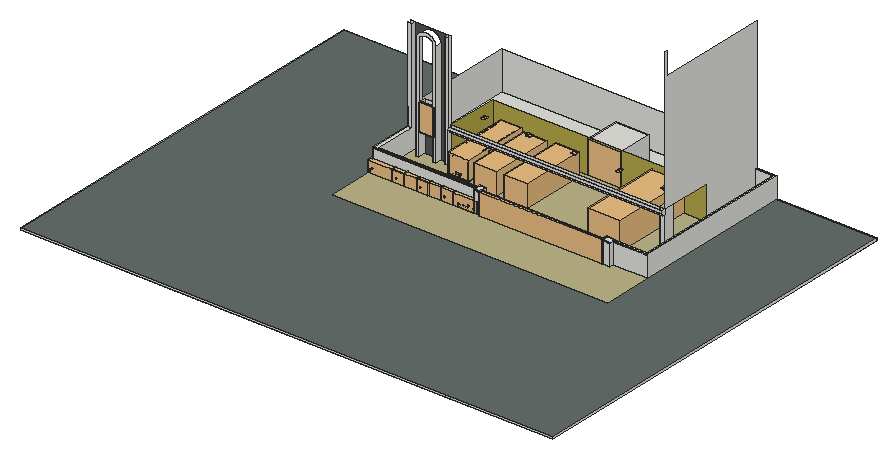
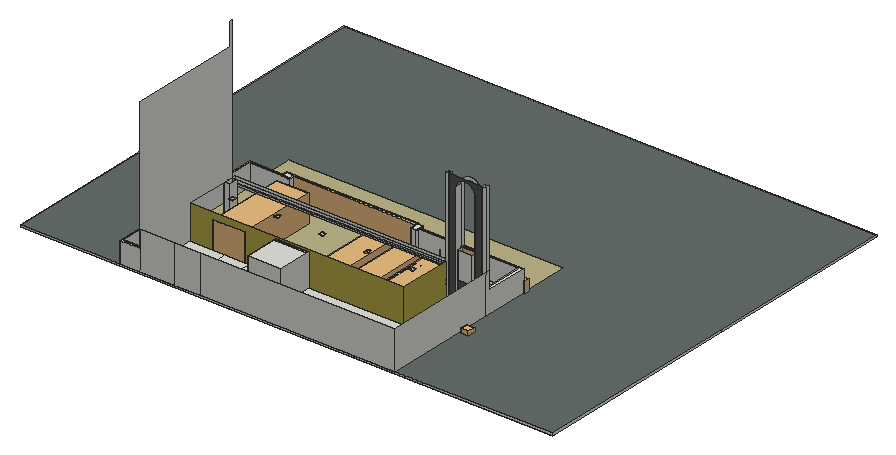
# SketchUp Ruby script. Lengths in inches.
U = 1.inch
M = Sketchup.active_model
def pt(a) = Geom::Point3d.new(a.map { |v| v * U })
def face(e, loops, mat)
  f = e.add_face(loops[0].map { |a| pt(a) })
  loops[1..].each { |l| e.add_face(l.map { |a| pt(a) }).erase! }
  f.material = f.back_material = mat if mat
  f
end
# faces: each face lists its corners as indices into pts; further lists are holes
def faces(e, pts, list, mat = nil) = list.each { |f| face(e, (f[0].is_a?(Array) ? f : [f]).map { |l| l.map { |i| pts[i] } }, mat) }
# xy, xz, yz: faces in a plane at the given z, y or x. An outline is a flat list of corners, or four numbers for a rectangle; further outlines are holes
def ring(l) = l.size == 4 ? [[l[0], l[1]], [l[2], l[1]], [l[2], l[3]], [l[0], l[3]]] : l.each_slice(2).to_a
def flat(e, list, mat, &to3) = list.each { |f| face(e, (f[0].is_a?(Array) ? f : [f]).map { |l| ring(l).map { |u, v| to3.(u, v) } }, mat) }
def xy(e, z, list, mat = nil) = flat(e, list, mat) { |x, y| [x, y, z] }
def xz(e, y, list, mat = nil) = flat(e, list, mat) { |x, z| [x, y, z] }
def yz(e, x, list, mat = nil) = flat(e, list, mat) { |y, z| [x, y, z] }
def lines(e, pts, list) = list.each { |a, b| e.add_line(pt(pts[a]), pt(pts[b])) }
# prism: a flat outline (further loops are holes) pulled along v
def prism(e, loops, v, mat = nil)
  f = face(e, loops, mat); d = Geom::Vector3d.new(v.map { |x| x * U })
  f.pushpull(f.normal.samedirection?(d) ? d.length : -d.length)
end
def box(e, o, s, mat = nil) = prism(e, [[o, [o[0] + s[0], o[1], o[2]], [o[0] + s[0], o[1] + s[1], o[2]], [o[0], o[1] + s[1], o[2]]]], [0, 0, s[2]], mat)
def at(x, y, z, deg = 0) = Geom::Transformation.translation(pt([x, y, z])) * Geom::Transformation.rotation(ORIGIN, Z_AXIS, deg.degrees)
def axes(o, x, y, z) = Geom::Transformation.new([*x, 0, *y, 0, *z, 0, *pt(o).to_a, 1])
def part(name) = M.definitions.add(name)
# library, detail: a bought-in or finely detailed component or shape, given as its bounding box
def library(name, o, s) = part(name).tap { |d| box(d.entities, o, s) }
def detail(e, o, s) = box(e.add_group.entities, o, s)
def put(e, d, t, mat = nil) = e.add_instance(d, t).tap { |i| i.material = mat if mat }
def group(e, t, mat = nil) = e.add_group.tap { |g| g.transformation = t; g.material = mat if mat }.entities
root = M.entities
M.materials.add("LCD Screen").color = [40, 40, 51]
M.materials.add("[0046_Gold]").color = [181, 168, 73]
M.materials.add("[0133_Gray]").color = [128, 128, 128]
M.materials.add("[Color M06]").color = [86, 86, 86]
M.materials.add("[Slate]").color = [102, 110, 108]
M.materials.add("[Tile Ceramic Natural]").color = [189, 180, 134]
c1 = library("Dome Light",[-12,-12,0],[24,24,12])
c2 = library("PINTU 7 YA",[-35.83,-0.24,0],[35.83,6.78,80.71])
c3 = library("CONG SAT 04",[0,-1.63,0],[141.97,7.2,115.26])
c4 = library("Group\#88",[0,0,0],[56.8,25.91,35.15])
c5 = library("bmw m6",[0,0,0],[74.56,175.18,49.66])
c6 = library("araç",[-7.9,-14.14,0],[84.07,190.26,56.29])
c7 = library("DLP_alu",[-32.56,-4.95,28.46],[3.03,21.46,11.47])
c8 = part("DLP_cbs")
p = [[-36.52,23.4375,42.01],[-35.11,24.24,42.09],[-35.4,24.125,40.43],[-36.74,23.36,40.52],[-38.26,22.15,41.875],[-38.47,22.06,40.56],
  [-40.67,17.9,41.7],[-40.67,18.91,41.7],[-40.8,18.84,40.61],[-40.8,17.85,40.61],[-40.375,20,41.73],[-40.53,19.93,40.61],
  [-39.86,20.78,41.76],[-40.03,20.71,40.6]]
faces(c8.entities,p,[[0,1,2,3],[4,0,3,5],[6,7,8,9],[8,7,10],[11,8,10],[11,10,12],[13,11,12],[13,12,4],
  [5,13,4]],"[0133_Gray]")
c9 = library("DLP_chr",[-40.43,-8.43,15.5],[8.39,45.84,28.21])
c10 = library("DLP_gum",[-40.55,-8.34,12.92],[10.79,44.66,30.87])
c11 = library("DLP_lak",[-40.9,-8.24,11.52],[10.21,45.77,32.59])
c12 = library("DLP_skl",[-40.84,-9.76,38.62],[15.44,35.5,13.42])
c13 = library("DLP_tex",[-32.23,-4.24,14.11],[3.7,37.66,28.64])
c14 = library("DLZ_alu",[-32.64,-45.42,32.17],[3.13,26.43,8.08])
c15 = library("DLZ_chr",[-36.26,-50.38,17.1875],[5.37,44.24,23.07])
c16 = library("DLZ_gum",[-35.53,-50.63,13.6],[7.69,42.37,33.49])
c17 = library("DLZ_lak",[-36.74,-50.79,12.27],[6.11,44.87,27.25])
c18 = part("DLZ_skl")
p = [[-31.25,-30.73,40.37],[-31.5,-19.9,40.27],[-30.59,-48.22,40.18],[-30.92,-40.72,40.33],[-26.94,-12.67,49.97],[-25.41,-12.96,52.02],
  [-28.875,-12.22,46.74],[-30.54,-11.73,43.16],[-31.64,-11.31,40.09],[-31.8,-11.31,40.09]]
lines(c18.entities,p,[[0,1],[2,3],[3,0],[4,5],[6,4],[7,6],[1,8],[8,7],[8,9]])
detail(c18.entities,[-31.8,-48.22,40.09],[6.39,36.91,11.93])
c19 = library("DLZ_t",[-31.625,-44.63,14.78],[3.09,34.76,25.59])
c20 = library("DPP_alu",[29.53,-4.95,28.46],[3.03,21.46,11.47])
c21 = library("DPP_tex",[28.53,-4.24,14.11],[3.7,37.66,28.64])
c22 = library("Int_tex",[-31.25,-73.91,8.87],[62.5,119.46,45.3])
c23 = library("Kar_alu",[-29.72,81.17,25.34],[59.44,2.6,2.71])
c24 = library("Kar_cbs",[-32.74,-96.83,15.58],[65.48,186.26,20.5])
c25 = library("Kar_chr",[-36.16,-97.14,11.15],[72.32,193.86,41.64])
c26 = library("Kar_gum",[-36.56,-96.93,5.72],[73.12,192.75,46.42])
c27 = library("Kar_lak",[7.38,4.29,6.91],[74.38,195.36,48.89])
c28 = library("Kar_sbs",[-32.72,-92.46,24.22],[65.44,182.04,10.46])
c29 = library("Kar_skl",[-29.75,-104.29,14.29],[59.5,202.2,49.68])
c30 = library("Kar_tex",[-32.74,-92.93,9.48],[65.48,189.57,42.88])
c31 = library("Vol_tex",[-22.45,16.21,27.51],[14.96,7.24,13.71])
c32 = library("Wheels",[0,0,0],[9.18,26.12,26.12])
c33 = library("Brembo",[0,-5.36,-7],[3.52,47.83,47.82])
c34 = part("skp97F5")
put(c34.entities,c7,axes([39.67,109.0625,-0.73],[-0.89467,0,0],[0,-1.07561,0],[0,0,1.21635]))
put(c34.entities,c8,axes([39.67,109.0625,-0.73],[-0.89467,0,0],[0,-1.07561,0],[0,0,1.21635]))
put(c34.entities,c9,axes([39.67,109.0625,-0.73],[-0.89467,0,0],[0,-1.07561,0],[0,0,1.21635]))
put(c34.entities,c10,axes([39.67,109.0625,-0.73],[-0.89467,0,0],[0,-1.07561,0],[0,0,1.21635]))
put(c34.entities,c11,axes([39.67,109.0625,-0.73],[-0.89467,0,0],[0,-1.07561,0],[0,0,1.21635]))
put(c34.entities,c12,axes([39.67,109.0625,-0.73],[-0.89467,0,0],[0,-1.07561,0],[0,0,1.21635]))
put(c34.entities,c13,axes([39.67,109.0625,-0.73],[-0.89467,0,0],[0,-1.07561,0],[0,0,1.21635]))
put(c34.entities,c14,axes([39.67,109.0625,-0.73],[-0.89467,0,0],[0,-1.07561,0],[0,0,1.21635]))
put(c34.entities,c15,axes([39.67,109.0625,-0.73],[-0.89467,0,0],[0,-1.07561,0],[0,0,1.21635]))
put(c34.entities,c16,axes([39.67,109.0625,-0.73],[-0.89467,0,0],[0,-1.07561,0],[0,0,1.21635]))
put(c34.entities,c17,axes([39.67,109.0625,-0.73],[-0.89467,0,0],[0,-1.07561,0],[0,0,1.21635]))
put(c34.entities,c18,axes([39.67,109.0625,-0.73],[-0.89467,0,0],[0,-1.07561,0],[0,0,1.21635]))
put(c34.entities,c19,axes([39.67,109.0625,-0.73],[-0.89467,0,0],[0,-1.07561,0],[0,0,1.21635]))
put(c34.entities,c20,axes([39.67,109.0625,-0.73],[-0.89467,0,0],[0,-1.07561,0],[0,0,1.21635]))
put(c34.entities,c21,axes([39.67,109.0625,-0.73],[-0.89467,0,0],[0,-1.07561,0],[0,0,1.21635]))
put(c34.entities,c22,axes([39.67,109.0625,-0.73],[-0.89467,0,0],[0,-1.07561,0],[0,0,1.21635]))
put(c34.entities,c23,axes([39.67,109.0625,-0.73],[-0.89467,0,0],[0,-1.07561,0],[0,0,1.21635]))
put(c34.entities,c24,axes([39.67,109.0625,-0.73],[-0.89467,0,0],[0,-1.07561,0],[0,0,1.21635]))
put(c34.entities,c25,axes([39.67,109.0625,-0.73],[-0.89467,0,0],[0,-1.07561,0],[0,0,1.21635]))
put(c34.entities,c26,axes([39.67,109.0625,-0.73],[-0.89467,0,0],[0,-1.07561,0],[0,0,1.21635]))
put(c34.entities,c27,axes([0,0,0],[0.89,0,0],[0,1.07,0],[0,0,1.21]))
put(c34.entities,c28,axes([39.67,109.0625,-0.73],[-0.89467,0,0],[0,-1.07561,0],[0,0,1.21635]))
put(c34.entities,c29,at(39.67,109.0625,-0.73,180))
put(c34.entities,c30,axes([39.67,109.0625,-0.73],[-0.89467,0,0],[0,-1.07561,0],[0,0,1.21635]))
put(c34.entities,c31,axes([39.67,109.0625,-0.73],[-0.89467,0,0],[0,-1.07561,0],[0,0,1.21635]))
put(c34.entities,c32,axes([71.86,57.12,0],[-0.89,0,0],[0,-1.07,0],[0,0,1.21]))
put(c34.entities,c32,axes([72.42,178.23,0],[-0.89,0,0],[0,-1.07,0],[0,0,1.21]))
put(c34.entities,c32,axes([7.48,29.17,0],[0.89,0,0],[0,1.07,0],[0,0,1.21]))
put(c34.entities,c32,axes([6.91,150.28,0],[0.89,0,0],[0,1.07,0],[0,0,1.21]))
put(c34.entities,c12,axes([39.67,109.0625,-0.73],[0.89467,0,0],[0,-1.07561,0],[0,0,1.21635]))
put(c34.entities,c9,axes([39.67,109.0625,-0.73],[0.89467,0,0],[0,-1.07561,0],[0,0,1.21635]))
put(c34.entities,c11,axes([39.67,109.0625,-0.73],[0.89467,0,0],[0,-1.07561,0],[0,0,1.21635]))
put(c34.entities,c10,axes([39.67,109.0625,-0.73],[0.89467,0,0],[0,-1.07561,0],[0,0,1.21635]))
put(c34.entities,c15,axes([39.67,109.0625,-0.73],[0.89467,0,0],[0,-1.07561,0],[0,0,1.21635]))
put(c34.entities,c16,axes([39.67,109.0625,-0.73],[0.89467,0,0],[0,-1.07561,0],[0,0,1.21635]))
put(c34.entities,c17,axes([39.67,109.0625,-0.73],[0.89467,0,0],[0,-1.07561,0],[0,0,1.21635]))
put(c34.entities,c18,axes([39.67,109.0625,-0.73],[0.89467,0,0],[0,-1.07561,0],[0,0,1.21635]))
put(c34.entities,c19,axes([39.67,109.0625,-0.73],[0.89467,0,0],[0,-1.07561,0],[0,0,1.21635]))
put(c34.entities,c8,axes([39.67,109.0625,-0.73],[0.89467,0,0],[0,-1.07561,0],[0,0,1.21635]))
put(c34.entities,c14,axes([39.67,109.0625,-0.73],[0.89467,0,0],[0,-1.07561,0],[0,0,1.21635]))
put(c34.entities,c33,axes([68.85,165.18,4.4],[0.33559,0,0],[0,-0.29793,0.30765],[0,0.27205,0.33692]))
put(c34.entities,c33,axes([67.92,44.125,3.73],[0.35533,0,0],[0,-0.31546,0.32574],[0,0.28806,0.35674]))
put(c34.entities,c33,axes([11.41,44.125,3.73],[-0.35533,0,0],[0,-0.31546,0.32574],[0,0.28806,0.35674]))
put(c34.entities,c33,axes([10.49,165.18,4.4],[-0.33559,0,0],[0,-0.29793,0.30765],[0,0.27205,0.33692]))
c35 = part("Mercedes-Benz CLS 350 CDI W218 2012")
put(c35.entities,c34,at(0,0,0))
c36 = part("2011 Mercedes-Benz CLS550 4Matic")
put(c36.entities,c35,at(0,0,0))
c37 = library("Poulsen_Ballerup.skp\#1",[-1.79,-1.87,-0.84],[3.58,3.74,0.84])
c38 = library("Poulsen_Ballerup.skp",[-1.79,-1.87,-0.84],[3.58,3.74,0.84])
c39 = part("araba")
put(c39.entities,c36,at(0,0,0))
put(c39.entities,c37,axes([64.93,19.18,32.04],[1,0,0],[0,0,-1],[0,1,0]))
put(c39.entities,c38,axes([14.56,19.07,32.04],[1,0,0],[0,0,-1],[0,1,0]))
c40 = library("plaka",[1.7,0.67,0],[15.75,0.09,3.9375])
c41 = part("MERCEDES LIGHT")
put(c41.entities,c39,at(9.53,109.0625,0.73,-180),"LCD Screen")
put(c41.entities,c40,axes([-20.04,106.22,17.09],[-1.03,0,0],[0,-1.7548,0],[0,0,1.3673]))
put(c41.entities,c40,axes([-38.66,-100.89,37.09],[0.89,0,0],[0,1.03354,-0.31317],[0,0.27694,1.16877]))
c42 = part("cars")
put(c42.entities,c5,axes([-7.96,-11.59,0],[0.9968,0,0],[0,1.12927,0],[0,0,1.35817]))
put(c42.entities,c6,axes([95.6,3.14,0],[0.89,0,0],[0,1.07,0],[0,0,1.21]))
put(c42.entities,c41,at(-86.89,94.34,0,180))
c43 = library("RR Phanton",[0,0,0],[8.78,23.57,7.05])
c44 = library("Lamp Ceiling 114-44",[-1.26,-1.26,-3.9375],[2.52,2.52,3.9375])
c45 = library("Group\#12",[0,0,0],[48.03,6.47,83.79])
c46 = library("Tlon Light 1950 Ceiling 152 010",[-38.39,-38.39,-3.78],[76.78,76.78,3.41])
xy(root,-1.49,[[0,0,497.625,610.25],[497.625,0,1362.625,610.25],[1362.625,0,1677.875,610.25],[0,610.25,497.625,1276.1875],[497.625,610.25,1362.625,1276.1875],
  [1362.625,610.25,1677.875,1276.1875]])
xy(root,4.51,[[825.33,756.0625,842.33,756.0625,842.33,780.51,827.33,780.51,827.33,773.51,510,773.51,510,916.1875,497.625,916.1875,497.625,768.0625,825.33,768.0625],[[497.625,756.0625,825.33,768.0625],[499.24,757.68,823.72,766.45]],[1229.84,756.0625,1253.84,756.0625,1253.84,768.0625,1362.625,768.0625,1362.625,1276.1875,1299.8125,1276.1875,1299.8125,1270.1875,1356.5625,1270.1875,1356.5625,773.51,1229.84,773.51],[499.24,757.68,823.72,766.45],[533.1875,893.4375,541.1875,893.4375,541.1875,916.1875,586.375,916.1875,586.375,893.4375,594.375,893.4375,594.375,916.1875,624.25,916.1875,624.25,1080.1875,926.14,1080.1875,926.14,1190.125,1030.58,1190.125,1030.58,1080.1875,1112.75,1080.1875,1112.75,1276.1875,497.625,1276.1875,497.625,916.1875,533.1875,916.1875],
  [616.25,904.1875,624.25,916.1875],[1112.75,1080.1875,1189.1875,1276.1875],[1189.1875,1080.1875,1299.8125,1276.1875]])
xy(root,4.51,[[0,0,1677.875,0,1677.875,1276.1875,1362.625,1276.1875,1362.625,610.25,497.625,610.25,497.625,1276.1875,0,1276.1875]],"[Slate]")
xy(root,4.51,[[[497.625,610.25,1362.625,610.25,1362.625,768.0625,1253.84,768.0625,1253.84,756.0625,1229.84,756.0625,1229.84,773.51,1356.5625,773.51,1356.5625,1270.1875,1299.8125,1270.1875,1299.8125,1080.1875,1030.58,1080.1875,1030.58,1190.125,926.14,1190.125,926.14,1080.1875,624.25,1080.1875,624.25,904.1875,616.25,904.1875,616.25,916.1875,594.375,916.1875,594.375,893.4375,586.375,893.4375,586.375,916.1875,541.1875,916.1875,541.1875,893.4375,533.1875,893.4375,533.1875,916.1875,510,916.1875,510,773.51,827.33,773.51,827.33,780.51,842.33,780.51,842.33,756.0625,497.625,756.0625],[1281.875,916.1875,1299.8125,945.21]]],"[Tile Ceramic Natural]")
xy(root,16.51,[[[497.625,756.0625,825.33,768.0625],[499.24,757.68,823.72,766.45]]])
xy(root,68.76,[[497.625,767.5625,825.33,768.0625]])
xy(root,69.77,[[1253.84,767.5625,1254.84,768.0625],[1254.84,767.5625,1362.625,768.0625]])
xy(root,70.77,[[1228.84,755.0625,1254.84,756.0625],[824.83,755.5625,842.83,756.0625],[824.83,756.0625,825.33,767.5625],[825.33,756.0625,825.33,767.5625,824.83,767.5625,824.83,773.51,827.33,773.51,827.33,780.51,842.33,780.51,842.33,756.0625],[842.33,756.0625,842.83,780.51],
  [1228.84,756.0625,1229.84,774.51],[1229.84,756.0625,1229.84,773.51,1254.84,773.51,1254.84,767.5625,1253.84,767.5625,1253.84,756.0625],[1253.84,756.0625,1254.84,767.5625],[497.625,767.5625,824.83,767.5625,824.83,773.51,510,773.51,510,904.1875,497.625,904.1875],[1254.84,767.5625,1362.625,767.5625,1362.625,1276.1875,1299.8125,1276.1875,1299.8125,1270.1875,1356.5625,1270.1875,1356.5625,773.51,1254.84,773.51],
  [824.83,773.51,827.33,780.51],[1229.84,773.51,1254.84,774.51]])
xy(root,72.52,[[824.83,755.5625,842.83,780.51]])
xy(root,72.9,[[1228.84,755.0625,1254.84,774.51]])
xy(root,73.72,[[541.1875,893.4375,586.375,916.1875]])
xy(root,74.52,[[541.1875,893.4375,586.375,916.1875]])
xy(root,96.45,[[624.25,908.4375,1299.8125,916.1875]])
xy(root,104.51,[[624.25,904.1875,1299.8125,908.4375]])
xy(root,106.14,[[926.14,1080.1875,1030.58,1190.125]])
xz(root,0,[[0,-1.49,1362.625,4.51],[1362.625,-1.49,1677.875,4.51]])
xz(root,755.0625,[[1228.84,70.77,1254.84,72.9]])
xz(root,755.5625,[[824.83,70.77,842.83,72.52]])
xz(root,756.0625,[[497.625,4.51,825.33,16.51],[825.33,4.51,842.33,70.77],[1229.84,4.51,1253.84,70.77]])
xz(root,757.68,[[499.24,4.51,823.72,16.51]])
xz(root,766.45,[[499.24,4.51,823.72,16.51]])
xz(root,767.5625,[[497.625,68.76,825.33,70.77],[1253.84,69.77,1362.625,70.77]])
xz(root,768.0625,[[497.625,4.51,825.33,16.51],[1253.84,4.51,1362.625,69.77],[497.625,16.51,825.33,68.76]])
xz(root,773.51,[[510,4.51,827.33,70.77],[1229.84,4.51,1356.5625,70.77]])
xz(root,774.51,[[1228.84,70.77,1254.84,72.9]])
xz(root,780.51,[[827.33,4.51,842.33,70.77],[824.83,70.77,842.83,72.52]])
xz(root,893.4375,[[533.1875,4.51,541.1875,4.51,541.1875,342.21,541.625,342.7,542.77,343.84,543.97,344.92,545.23,345.93,546.54,346.88,547.9,347.76,549.3,348.5625,550.74,349.29,552.22,349.95,553.73,350.52,555.26,351.02,556.82,351.43,558.41,351.77,560,352.02,561.61,352.18,563.22,352.27,564.84,352.26,566.45,352.18,568.06,352,569.66,351.75,571.24,351.41,572.8,350.99,574.33,350.49,575.84,349.9,577.3125,349.24,578.75,348.51,580.15,347.7,581.5,346.82,582.81,345.86,584.0625,344.84,585.26,343.76,586.375,342.64,587,342.64,587,241.08,586.375,241.08,586.375,4.51,594.375,4.51,594.375,333.47,594.14,334.98,593.81,336.56,593.39,338.12,592.89,339.66,592.32,341.17,591.66,342.65,590.93,344.09,590.125,345.49,589.25,346.84,588.3,348.15,587.29,349.41,586.21,350.61,585.07,351.76,583.87,352.84,582.61,353.86,581.31,354.8125,579.96,355.7,578.56,356.51,577.12,357.24,575.64,357.9,574.14,358.48,572.6,358.99,571.04,359.41,569.46,359.75,567.86,360,566.26,360.17,564.64,360.26,563.03,360.26,561.41,360.18,559.81,360.02,558.21,359.77,556.63,359.43,555.07,359.02,553.53,358.52,552.02,357.94,550.54,357.29,549.1,356.56,547.7,355.75,546.34,354.875,545.04,353.93,543.78,352.91,542.58,351.83,541.43,350.69,540.35,349.49,539.33,348.24,538.375,346.93,537.49,345.58,536.68,344.18,535.95,342.74,535.29,341.27,534.7,339.76,534.2,338.23,533.78,336.67,533.44,335.09,533.1875,333.49],[541.1875,73.72,586.375,74.52]])
xz(root,904.1875,[[616.25,4.51,624.25,364.51],[497.625,70.77,510,364.51],[624.25,104.51,1299.8125,112.51]])
xz(root,908.4375,[[624.25,96.45,1299.8125,104.51]])
xz(root,916.1875,[[497.625,4.51,510,364.51],[616.25,4.51,624.25,364.51],[1281.875,4.51,1299.8125,96.45],[541.1875,74.52,586.375,158.17],[624.25,96.45,1281.875,100.51],
  [1281.875,96.45,1299.8125,100.51],[624.25,100.51,1281.875,104.51],[1281.875,100.51,1299.8125,104.51],[624.25,104.51,1281.875,112.51],[1281.875,104.51,1299.8125,112.51]])
xz(root,916.1875,[[510,4.51,533.1875,4.51,533.1875,333.49,533.44,335.09,533.78,336.67,534.2,338.23,534.7,339.76,535.29,341.27,535.95,342.74,536.68,344.18,537.49,345.58,538.375,346.93,539.33,348.24,540.35,349.49,541.43,350.69,542.58,351.83,543.78,352.91,545.04,353.93,546.34,354.875,547.7,355.75,549.1,356.56,550.54,357.29,552.02,357.94,553.53,358.52,555.07,359.02,556.63,359.43,558.21,359.77,559.81,360.02,561.41,360.18,563.03,360.26,564.64,360.26,566.26,360.17,567.86,360,569.46,359.75,571.04,359.41,572.6,358.99,574.14,358.48,575.64,357.9,577.12,357.24,578.56,356.51,579.96,355.7,581.31,354.8125,582.61,353.86,583.87,352.84,585.07,351.76,586.21,350.61,587.29,349.41,588.3,348.15,589.25,346.84,590.125,345.49,590.93,344.09,591.66,342.65,592.32,341.17,592.89,339.66,593.39,338.12,593.81,336.56,594.14,334.98,594.375,333.47,594.39,333.38,594.56,331.77,594.64,330.16,594.63,328.54,594.55,326.93,594.46,326.15,594.375,326.72,594.375,333.47,594.39,333.38,594.56,331.77,594.64,330.16,594.63,328.54,594.55,326.93,594.46,326.15,594.375,325.32,594.375,4.51,616.25,4.51,616.25,364.51,510,364.51],[541.1875,4.51,586.375,73.72]],"[Color M06]")
xz(root,945.21,[[1281.875,4.51,1299.8125,112.51]])
xz(root,1080.1875,[[624.25,4.51,926.14,4.51,926.14,106.14,1030.58,106.14,1030.58,4.51,1299.8125,4.51,1299.8125,112.51,624.25,112.51]],"[0046_Gold]")
xz(root,1190.125,[[926.14,4.51,1030.58,106.14]])
xz(root,1270.1875,[[1299.8125,4.51,1356.5625,70.77]])
xz(root,1276.1875,[[0,-1.49,497.625,4.51],[497.625,-1.49,1362.625,4.51],[1362.625,-1.49,1677.875,4.51],[497.625,4.51,1112.75,124.51],[1112.75,4.51,1189.1875,124.51],
  [1189.1875,4.51,1299.8125,124.51],[1299.8125,4.51,1362.625,70.77]])
yz(root,0,[[0,-1.49,610.25,4.51],[610.25,-1.49,1276.1875,4.51]])
yz(root,497.625,[[756.0625,4.51,768.0625,16.51],[768.0625,4.51,768.0625,68.76,767.5625,68.76,767.5625,70.77,904.1875,70.77,904.1875,124.51,916.1875,124.51,916.1875,4.51],[916.1875,4.51,1276.1875,124.51]])
yz(root,499.24,[[757.68,4.51,766.45,16.51]])
yz(root,510,[[773.51,4.51,916.1875,4.51,916.1875,364.51,904.1875,364.51,904.1875,70.77,773.51,70.77]])
yz(root,533.1875,[[893.4375,4.51,916.1875,333.49]])
yz(root,541.1875,[[893.4375,4.51,916.1875,73.72],[893.4375,74.52,916.1875,158.17]])
yz(root,586.375,[[893.4375,4.51,916.1875,73.72],[893.4375,74.52,916.1875,158.17]])
yz(root,594.375,[[893.4375,4.51,916.1875,333.47]])
yz(root,616.25,[[904.1875,4.51,916.1875,364.51]])
yz(root,624.25,[[904.1875,4.51,916.1875,4.51,916.1875,96.45,908.4375,96.45,908.4375,104.51,904.1875,104.51],[908.4375,96.45,916.1875,100.51],[908.4375,100.51,916.1875,104.51]])
yz(root,624.25,[[916.1875,4.51,1080.1875,112.51]],"[0046_Gold]")
yz(root,823.72,[[757.68,4.51,766.45,16.51]])
yz(root,824.83,[[755.5625,70.77,780.51,72.52]])
yz(root,825.33,[[756.0625,4.51,768.0625,16.51],[756.0625,16.51,756.0625,70.77,767.5625,70.77,767.5625,68.76,768.0625,68.76,768.0625,16.51]])
yz(root,827.33,[[773.51,4.51,780.51,70.77]])
yz(root,842.33,[[756.0625,4.51,780.51,70.77]])
yz(root,842.83,[[755.5625,70.77,780.51,72.52]])
yz(root,926.14,[[1080.1875,4.51,1190.125,106.14]])
yz(root,1030.58,[[1080.1875,4.51,1190.125,106.14]])
yz(root,1228.84,[[755.0625,70.77,774.51,72.9]])
yz(root,1229.84,[[756.0625,4.51,773.51,70.77]])
yz(root,1253.84,[[756.0625,4.51,768.0625,4.51,768.0625,69.77,767.5625,69.77,767.5625,70.77,756.0625,70.77]])
yz(root,1254.84,[[755.0625,70.77,768.0625,72.9],[768.0625,70.77,774.51,72.9]])
yz(root,1281.875,[[916.1875,4.51,945.21,112.51]])
yz(root,1299.8125,[[1080.1875,4.51,1270.1875,4.51,1270.1875,70.77,1276.1875,70.77,1276.1875,484.51,924.1875,484.51,924.1875,556.51,916.1875,556.51,916.1875,112.51,1080.1875,112.51],[916.1875,4.51,945.21,112.51],[908.4375,96.45,916.1875,96.45,916.1875,112.51,904.1875,112.51,904.1875,104.51,908.4375,104.51]])
yz(root,1356.5625,[[773.51,4.51,1270.1875,70.77]])
yz(root,1362.625,[[768.0625,4.51,1276.1875,4.51,1276.1875,70.77,767.5625,70.77,767.5625,69.77,768.0625,69.77]])
yz(root,1677.875,[[0,-1.49,1276.1875,4.51]])
put(root,c1,at(480.6,1010.22,4.51))
put(root,c2,axes([1030.41,1080.42,4.51],[2.90966,0,0],[0,0.96507,0],[0,0,1.26]))
put(root,c3,axes([842.83,756.0625,4.51],[2.74612,0,0],[0,1,0],[0,0,0.59006]))
put(root,c4,axes([492.32,754.77,4.51],[1.998,0,0],[0,0.6,0],[0,0,1]))
put(root,c42,at(749.52,870.2,4.51))
put(root,c4,axes([568.52,755.2,4.51],[1.998,0,0],[0,0.6,0],[0,0,1]))
put(root,c4,axes([644.72,755.63,4.51],[1.998,0,0],[0,0.6,0],[0,0,1]))
put(root,c4,axes([720.93,756.0625,4.51],[1.998,0,0],[0,0.6,0],[0,0,1]))
put(root,c43,axes([1126.54,830.07,4.51],[11.48,0,0],[0,10.61264,0],[0,0,12.3372]))
put(root,c44,axes([808.65,757.51,16.4375],[-1,0,0],[0,1,0],[0,0,-1]))
put(root,c44,axes([733.02,757.46,16.46],[-1,0,0],[0,1,0],[0,0,-1]))
put(root,c44,axes([657.4,757.42,16.48],[-1,0,0],[0,1,0],[0,0,-1]))
put(root,c44,axes([581.77,757.37,16.49],[-1,0,0],[0,1,0],[0,0,-1]))
put(root,c44,axes([506.15,757.32,16.51],[-1,0,0],[0,1,0],[0,0,-1]))
put(root,c45,at(540.48,893.4375,74.52))
put(root,c46,axes([664.85,996.9,112.62],[0.16,0,0],[0,0.16,0],[0,0,0.16]))
put(root,c46,axes([806.6,996.9,112.62],[0.16,0,0],[0,0.16,0],[0,0,0.16]))
put(root,c46,axes([948.35,996.9,112.62],[0.16,0,0],[0,0.16,0],[0,0,0.16]))
put(root,c46,axes([1090.1,996.9,112.62],[0.16,0,0],[0,0.16,0],[0,0,0.16]))
put(root,c46,axes([1231.85,996.9,112.62],[0.16,0,0],[0,0.16,0],[0,0,0.16]))
